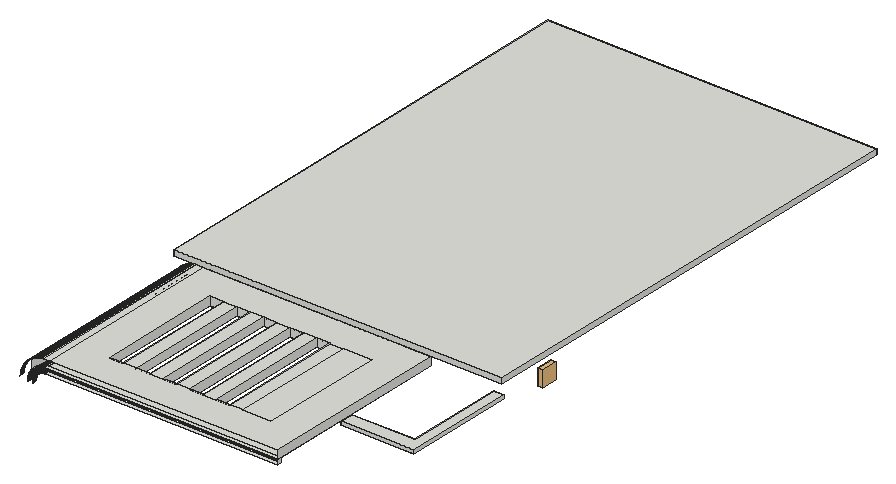
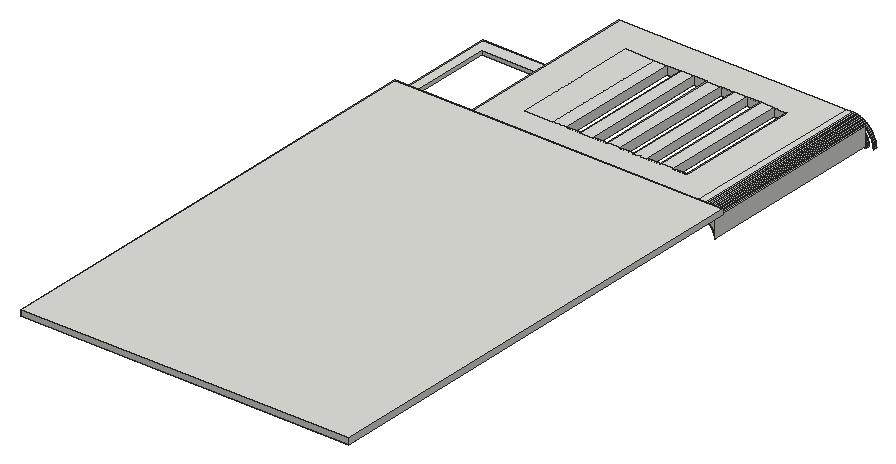
# SketchUp Ruby script. Lengths in inches.
U = 1.inch
M = Sketchup.active_model
def pt(a) = Geom::Point3d.new(a.map { |v| v * U })
def face(e, loops, mat)
  f = e.add_face(loops[0].map { |a| pt(a) })
  loops[1..].each { |l| e.add_face(l.map { |a| pt(a) }).erase! }
  f.material = f.back_material = mat if mat
  f
end
# faces: each face lists its corners as indices into pts; further lists are holes
def faces(e, pts, list, mat = nil) = list.each { |f| face(e, (f[0].is_a?(Array) ? f : [f]).map { |l| l.map { |i| pts[i] } }, mat) }
# xy, xz, yz: faces in a plane at the given z, y or x. An outline is a flat list of corners, or four numbers for a rectangle; further outlines are holes
def ring(l) = l.size == 4 ? [[l[0], l[1]], [l[2], l[1]], [l[2], l[3]], [l[0], l[3]]] : l.each_slice(2).to_a
def flat(e, list, mat, &to3) = list.each { |f| face(e, (f[0].is_a?(Array) ? f : [f]).map { |l| ring(l).map { |u, v| to3.(u, v) } }, mat) }
def xy(e, z, list, mat = nil) = flat(e, list, mat) { |x, y| [x, y, z] }
def xz(e, y, list, mat = nil) = flat(e, list, mat) { |x, z| [x, y, z] }
def yz(e, x, list, mat = nil) = flat(e, list, mat) { |y, z| [x, y, z] }
def lines(e, pts, list) = list.each { |a, b| e.add_line(pt(pts[a]), pt(pts[b])) }
# prism: a flat outline (further loops are holes) pulled along v
def prism(e, loops, v, mat = nil)
  f = face(e, loops, mat); d = Geom::Vector3d.new(v.map { |x| x * U })
  f.pushpull(f.normal.samedirection?(d) ? d.length : -d.length)
end
def box(e, o, s, mat = nil) = prism(e, [[o, [o[0] + s[0], o[1], o[2]], [o[0] + s[0], o[1] + s[1], o[2]], [o[0], o[1] + s[1], o[2]]]], [0, 0, s[2]], mat)
def at(x, y, z, deg = 0) = Geom::Transformation.translation(pt([x, y, z])) * Geom::Transformation.rotation(ORIGIN, Z_AXIS, deg.degrees)
def axes(o, x, y, z) = Geom::Transformation.new([*x, 0, *y, 0, *z, 0, *pt(o).to_a, 1])
def part(name) = M.definitions.add(name)
# library, detail: a bought-in or finely detailed component or shape, given as its bounding box
def library(name, o, s) = part(name).tap { |d| box(d.entities, o, s) }
def detail(e, o, s) = box(e.add_group.entities, o, s)
def put(e, d, t, mat = nil) = e.add_instance(d, t).tap { |i| i.material = mat if mat }
def group(e, t, mat = nil) = e.add_group.tap { |g| g.transformation = t; g.material = mat if mat }.entities
root = M.entities
c1 = library("Agrupar\#12",[-0.01,0,0],[12.55,78.74,39.39])
xy(root,358,[[27.87,40.1875,282.03,44.1875]])
xy(root,363,[[27.87,40.1875,282.03,43.1875],[27.87,43.1875,282.03,44.1875],[[27.87,44.1875,282.03,250.1875],[156.5,76.1875,171.11,214.1875],[68.83,76.1875,83.4375,214.1875],[98.05,76.1875,112.66,214.1875],[127.28,76.1875,141.89,214.1875],[185.73,76.1875,200.34,214.1875]]])
xy(root,363.89,[[27.87,40.1875,282.03,43.1875]])
xy(root,372,[[25.95,40.1875,32.83,250.1875],[[32.83,40.1875,282.03,250.1875],[68.83,76.1875,246.03,214.1875]],[83.4375,76.1875,98.05,214.1875],[112.66,76.1875,127.28,214.1875],[141.89,76.1875,156.5,214.1875],
  [171.11,76.1875,185.73,214.1875],[200.34,76.1875,214.95,214.1875],[214.95,76.1875,246.03,214.1875]])
xz(root,44.1875,[[9,344.13,9,364.72,9.02,345.61,9.02,345.02,9.01,344.72]])
xz(root,76.1875,[[68.83,363,83.4375,372],[98.05,363,112.66,372],[127.28,363,141.89,372],[156.5,363,171.11,372],[185.73,363,200.34,372]])
xz(root,214.1875,[[68.83,363,83.4375,372],[98.05,363,112.66,372],[127.28,363,141.89,372],[156.5,363,171.11,372],[185.73,363,200.34,372]])
xz(root,250.1875,[[9.02,345.02,9.02,345.61,9,364.72,9,364.73,9.39,365.09,10.0625,365.66,10.75,366.21,11.45,366.73,12.17,367.24,12.9,367.72,13.65,368.18,14.41,368.61,15.1875,369.02,15.97,369.41,16.77,369.77,17.58,370.11,18.41,370.42,19.24,370.7,20.07,370.96,20.92,371.19,21.77,371.4,22.63,371.57,23.5,371.72,24.37,371.85,25.24,371.94,25.95,372,282.03,372,282.03,363,27.87,363,27.28,362.99,26.68,362.96,26.09,362.92,25.5,362.85,24.92,362.77,24.33,362.67,23.75,362.55,23.18,362.41,22.6,362.25,22.04,362.08,21.48,361.88,20.92,361.67,20.375,361.45,19.83,361.2,19.3,360.94,18.78,360.67,18.26,360.37,17.76,360.0625,17.26,359.74,16.78,359.4,16.3,359.04,15.84,358.67,15.39,358.28,14.95,357.89,14.11,357.05,13.72,356.61,13.33,356.16,12.96,355.7,12.6,355.22,12.26,354.74,11.9375,354.24,11.63,353.74,11.33,353.22,11.06,352.7,10.8,352.17,10.55,351.625,10.33,351.08,10.12,350.52,9.92,349.96,9.75,349.4,9.59,348.82,9.45,348.25,9.33,347.67,9.23,347.08,9.15,346.5,9.08,345.91,9.04,345.32]])
yz(root,9,[[44.1875,364.72,250.1875,364.73]])
yz(root,9.02,[[44.1875,345.02,250.1875,345.61]])
yz(root,68.83,[[76.1875,363,214.1875,372]])
yz(root,83.4375,[[76.1875,363,214.1875,372]])
yz(root,98.05,[[76.1875,363,214.1875,372]])
yz(root,112.66,[[76.1875,363,214.1875,372]])
yz(root,127.28,[[76.1875,363,214.1875,372]])
yz(root,141.89,[[76.1875,363,214.1875,372]])
yz(root,156.5,[[76.1875,363,214.1875,372]])
yz(root,171.11,[[76.1875,363,214.1875,372]])
yz(root,185.73,[[76.1875,363,214.1875,372]])
yz(root,200.34,[[76.1875,363,214.1875,372]])
yz(root,282.03,[[40.1875,358,44.1875,363],[43.1875,363,250.1875,363,250.1875,372,40.1875,372,40.1875,363.89,43.1875,363.89]])
p = [[8.12,40.1875,344.75],[8.11,40.1875,344.13],[8.11,43.1875,344.13],[8.12,43.1875,344.75],[9.01,40.1875,344.72],[9,40.1875,344.13],
  [9,43.1875,344.13],[9.01,43.1875,344.72],[14.01,40.1875,344.57],[14,40.1875,344.13],[14,44.1875,344.13],[14.01,44.1875,344.57],
  [9.01,44.1875,344.72],[9,44.1875,344.13],[14.03,40.1875,345],[14.03,44.1875,345],[9.04,40.1875,345.32],[9.04,43.1875,345.32],
  [9.04,44.1875,345.32],[9.02,44.1875,345.02],[8.14,40.1875,345.37],[8.14,43.1875,345.37],[14.0625,40.1875,345.4375],[14.0625,44.1875,345.4375],
  [9.02,250.1875,345.02],[9.04,250.1875,345.32],[9.08,40.1875,345.91],[9.08,43.1875,345.91],[9.08,44.1875,345.91],[9.08,250.1875,345.91],
  [8.19,40.1875,345.99],[8.19,43.1875,345.99],[14.11,40.1875,345.87],[14.11,44.1875,345.87],[9.02,44.1875,345.61],[9,44.1875,364.72],
  [9,250.1875,364.72],[9.02,250.1875,345.61],[9.15,40.1875,346.5],[9.15,43.1875,346.5],[14.17,40.1875,346.3],[14.17,44.1875,346.3],
  [9.15,44.1875,346.5],[9.15,250.1875,346.5],[0,40.1875,346.05],[0.06,40.1875,346.76],[0.06,44.1875,346.76],[0,44.1875,346.05],
  [8.26,40.1875,346.61],[8.26,43.1875,346.61],[14.25,40.1875,346.73],[14.25,44.1875,346.73],[9.23,40.1875,347.08],[9.23,43.1875,347.08],
  [9.23,44.1875,347.08],[9.23,250.1875,347.08],[8.35,40.1875,347.22],[8.35,43.1875,347.22],[14.33,40.1875,347.16],[14.33,44.1875,347.16],
  [0.15,40.1875,347.63],[0.15,44.1875,347.63],[9.33,40.1875,347.67],[9.33,43.1875,347.67],[9.33,44.1875,347.67],[9.33,250.1875,347.67],
  [8.46,40.1875,347.83],[8.46,43.1875,347.83],[14.4375,40.1875,347.58],[14.4375,44.1875,347.58],[0.28,40.1875,348.5],[0.28,44.1875,348.5],
  [14.55,40.1875,348],[14.55,44.1875,348],[9.45,40.1875,348.25],[9.45,43.1875,348.25],[9.45,44.1875,348.25],[9.45,250.1875,348.25],
  [8.58,40.1875,348.44],[8.58,43.1875,348.44],[14.68,40.1875,348.42],[14.68,44.1875,348.42],[9.59,40.1875,348.82],[9.59,43.1875,348.82],
  [9.59,44.1875,348.82],[9.59,250.1875,348.82],[8.73,40.1875,349.05],[8.73,43.1875,349.05],[14.82,40.1875,348.83],[14.82,44.1875,348.83],
  [0.43,40.1875,349.37],[0.43,44.1875,349.37],[9.75,40.1875,349.4],[9.75,43.1875,349.4],[14.97,40.1875,349.24],[14.97,44.1875,349.24],
  [9.75,44.1875,349.4],[9.75,250.1875,349.4],[8.89,40.1875,349.64],[8.89,43.1875,349.64],[15.14,40.1875,349.64],[15.14,44.1875,349.64],
  [0.6,40.1875,350.23],[0.6,44.1875,350.23],[9.92,40.1875,349.96],[9.92,43.1875,349.96],[9.92,44.1875,349.96],[9.92,250.1875,349.96],
  [9.07,40.1875,350.24],[9.07,43.1875,350.24],[15.32,40.1875,350.04],[15.32,44.1875,350.04],[10.12,40.1875,350.52],[10.12,43.1875,350.52],
  [15.51,40.1875,350.43],[15.51,44.1875,350.43],[10.12,44.1875,350.52],[10.12,250.1875,350.52],[0.81,40.1875,351.08],[0.81,44.1875,351.08],
  [9.27,40.1875,350.83],[9.27,43.1875,350.83],[15.72,40.1875,350.8125],[15.72,44.1875,350.8125],[10.33,40.1875,351.08],[10.33,43.1875,351.08],
  [10.33,44.1875,351.08],[10.33,250.1875,351.08],[9.49,40.1875,351.41],[9.49,43.1875,351.41],[15.93,40.1875,351.19],[15.93,44.1875,351.19],
  [1.04,40.1875,351.93],[1.04,44.1875,351.93],[10.55,40.1875,351.625],[10.55,43.1875,351.625],[10.55,44.1875,351.625],[10.55,250.1875,351.625],
  [16.16,40.1875,351.5625],[16.16,44.1875,351.5625],[9.73,40.1875,351.98],[9.73,43.1875,351.98],[10.8,40.1875,352.17],[10.8,43.1875,352.17],
  [16.4,40.1875,351.93],[16.4,44.1875,351.93],[10.8,44.1875,352.17],[10.8,250.1875,352.17],[1.3,40.1875,352.76],[1.3,44.1875,352.76],
  [16.65,40.1875,352.28],[16.65,44.1875,352.28],[9.99,40.1875,352.55],[9.99,43.1875,352.55],[11.06,40.1875,352.7],[11.06,43.1875,352.7],
  [11.06,44.1875,352.7],[11.06,250.1875,352.7],[16.91,40.1875,352.63],[16.91,44.1875,352.63],[10.26,40.1875,353.1],[10.26,43.1875,353.1],
  [17.18,40.1875,352.97],[17.18,44.1875,352.97],[11.33,40.1875,353.22],[11.33,43.1875,353.22],[11.33,44.1875,353.22],[11.33,250.1875,353.22],
  [1.58,40.1875,353.59],[1.58,44.1875,353.59],[17.47,40.1875,353.3],[17.47,44.1875,353.3],[10.55,40.1875,353.65],[10.55,43.1875,353.65],
  [11.63,40.1875,353.74],[11.63,43.1875,353.74],[11.63,44.1875,353.74],[11.63,250.1875,353.74],[17.76,40.1875,353.625],[17.76,44.1875,353.625],
  [1.89,40.1875,354.42],[1.89,44.1875,354.42],[18.0625,40.1875,353.9375],[18.0625,44.1875,353.9375],[10.86,40.1875,354.19],[10.86,43.1875,354.19],
  [11.9375,40.1875,354.24],[11.9375,43.1875,354.24],[11.9375,44.1875,354.24],[11.9375,250.1875,354.24],[18.375,40.1875,354.24],[18.375,44.1875,354.24],
  [11.18,40.1875,354.72],[11.18,43.1875,354.72],[12.26,40.1875,354.74],[12.26,43.1875,354.74],[18.7,40.1875,354.53],[18.7,44.1875,354.53],
  [12.26,44.1875,354.74],[12.26,250.1875,354.74],[2.23,40.1875,355.23],[2.23,44.1875,355.23],[19.03,40.1875,354.82],[19.03,44.1875,354.82],
  [11.52,40.1875,355.24],[11.52,43.1875,355.24],[12.6,40.1875,355.22],[12.6,43.1875,355.22],[12.6,44.1875,355.22],[12.6,250.1875,355.22],
  [19.37,40.1875,355.09],[19.37,44.1875,355.09],[19.72,40.1875,355.35],[19.72,44.1875,355.35],[2.59,40.1875,356.03],[2.59,44.1875,356.03],
  [11.88,40.1875,355.75],[11.88,43.1875,355.75],[12.96,40.1875,355.7],[12.96,43.1875,355.7],[12.96,44.1875,355.7],[12.96,250.1875,355.7],
  [20.07,40.1875,355.6],[20.07,44.1875,355.6],[20.4375,40.1875,355.84],[20.4375,44.1875,355.84],[12.25,40.1875,356.24],[12.25,43.1875,356.24],
  [13.33,40.1875,356.16],[13.33,43.1875,356.16],[13.33,44.1875,356.16],[13.33,250.1875,356.16],[20.81,40.1875,356.07],[20.81,44.1875,356.07],
  [2.98,40.1875,356.8125],[2.98,44.1875,356.8125],[21.1875,40.1875,356.28],[21.1875,44.1875,356.28],[12.64,40.1875,356.73],[12.64,43.1875,356.73],
  [13.72,40.1875,356.61],[13.72,43.1875,356.61],[13.72,44.1875,356.61],[13.72,250.1875,356.61],[21.57,40.1875,356.49],[21.57,44.1875,356.49],
  [21.96,40.1875,356.68],[21.96,44.1875,356.68],[14.11,40.1875,357.05],[14.11,43.1875,357.05],[14.11,44.1875,357.05],[14.11,250.1875,357.05],
  [13.04,40.1875,357.2],[13.04,43.1875,357.2],[22.36,40.1875,356.86],[22.36,44.1875,356.86],[3.39,40.1875,357.59],[3.39,44.1875,357.59],
  [22.76,40.1875,357.03],[22.76,44.1875,357.03],[14.53,40.1875,357.47],[14.53,43.1875,357.47],[23.17,40.1875,357.18],[23.17,44.1875,357.18],
  [14.53,44.1875,357.47],[14.53,250.1875,357.47],[13.46,40.1875,357.66],[13.46,43.1875,357.66],[23.58,40.1875,357.32],[23.58,44.1875,357.32],
  [24,40.1875,357.45],[24,44.1875,357.45],[24.42,40.1875,357.5625],[24.42,44.1875,357.5625],[14.95,40.1875,357.89],[14.95,43.1875,357.89],
  [14.95,44.1875,357.89],[14.95,250.1875,357.89],[3.82,40.1875,358.35],[3.82,44.1875,358.35],[24.84,40.1875,357.67],[24.84,44.1875,357.67],
  [13.89,40.1875,358.11],[13.89,43.1875,358.11],[25.27,40.1875,357.75],[25.27,44.1875,357.75],[25.7,40.1875,357.83],[25.7,44.1875,357.83],
  [26.13,40.1875,357.89],[26.13,44.1875,357.89],[15.39,40.1875,358.28],[15.39,43.1875,358.28],[26.5625,40.1875,357.9375],[26.5625,44.1875,357.9375],
  [27,40.1875,357.97],[27,44.1875,357.97],[15.39,44.1875,358.28],[15.39,250.1875,358.28],[27.43,40.1875,357.99],[27.43,44.1875,357.99],
  [27.87,40.1875,358],[27.87,44.1875,358],[14.34,40.1875,358.54],[14.34,43.1875,358.54],[15.84,40.1875,358.67],[15.84,43.1875,358.67],
  [15.84,44.1875,358.67],[15.84,250.1875,358.67],[4.28,40.1875,359.1],[4.28,44.1875,359.1],[14.8,40.1875,358.96],[14.8,43.1875,358.96],
  [16.3,40.1875,359.04],[16.3,43.1875,359.04],[16.3,44.1875,359.04],[16.3,250.1875,359.04],[15.27,40.1875,359.36],[15.27,43.1875,359.36],
  [16.78,40.1875,359.4],[16.78,43.1875,359.4],[16.78,44.1875,359.4],[16.78,250.1875,359.4],[4.76,40.1875,359.83],[4.76,44.1875,359.83],
  [15.76,40.1875,359.75],[15.76,43.1875,359.75],[17.26,40.1875,359.74],[17.26,43.1875,359.74],[17.26,44.1875,359.74],[17.26,250.1875,359.74],
  [16.25,40.1875,360.12],[16.25,43.1875,360.12],[17.76,40.1875,360.0625],[17.76,43.1875,360.0625],[17.76,44.1875,360.0625],[17.76,250.1875,360.0625],
  [5.27,40.1875,360.55],[5.27,44.1875,360.55],[16.76,40.1875,360.48],[16.76,43.1875,360.48],[18.26,40.1875,360.37],[18.26,43.1875,360.37],
  [18.26,44.1875,360.37],[18.26,250.1875,360.37],[18.78,40.1875,360.67],[18.78,43.1875,360.67],[18.78,44.1875,360.67],[18.78,250.1875,360.67],
  [17.28,40.1875,360.82],[17.28,43.1875,360.82],[5.79,40.1875,361.25],[5.79,44.1875,361.25],[19.3,40.1875,360.94],[19.3,43.1875,360.94],
  [19.3,44.1875,360.94],[19.3,250.1875,360.94],[17.81,40.1875,361.14],[17.81,43.1875,361.14],[19.83,40.1875,361.2],[19.83,43.1875,361.2],
  [19.83,44.1875,361.2],[19.83,250.1875,361.2],[18.35,40.1875,361.45],[18.35,43.1875,361.45],[20.375,40.1875,361.45],[20.375,43.1875,361.45],
  [20.375,44.1875,361.45],[20.375,250.1875,361.45],[6.34,40.1875,361.9375],[6.34,44.1875,361.9375],[18.9,40.1875,361.74],[18.9,43.1875,361.74],
  [20.92,40.1875,361.67],[20.92,43.1875,361.67],[20.92,44.1875,361.67],[20.92,250.1875,361.67],[19.45,40.1875,362.01],[19.45,43.1875,362.01],
  [21.48,40.1875,361.88],[21.48,43.1875,361.88],[21.48,44.1875,361.88],[21.48,250.1875,361.88],[6.91,40.1875,362.61],[6.91,44.1875,362.61],
  [22.04,40.1875,362.08],[22.04,43.1875,362.08],[22.04,44.1875,362.08],[22.04,250.1875,362.08],[20.02,40.1875,362.27],[20.02,43.1875,362.27],
  [22.6,40.1875,362.25],[22.6,43.1875,362.25],[22.6,44.1875,362.25],[22.6,250.1875,362.25],[20.59,40.1875,362.51],[20.59,43.1875,362.51],
  [23.18,40.1875,362.41],[23.18,43.1875,362.41],[23.18,44.1875,362.41],[23.18,250.1875,362.41],[23.75,40.1875,362.55],[23.75,43.1875,362.55],
  [23.75,44.1875,362.55],[23.75,250.1875,362.55],[21.17,40.1875,362.73],[21.17,43.1875,362.73],[24.33,40.1875,362.67],[24.33,43.1875,362.67],
  [24.33,44.1875,362.67],[24.33,250.1875,362.67],[7.5,40.1875,363.26],[7.5,44.1875,363.26],[21.76,40.1875,362.93],[21.76,43.1875,362.93],
  [24.92,40.1875,362.77],[24.92,43.1875,362.77],[24.92,44.1875,362.77],[24.92,250.1875,362.77],[25.5,40.1875,362.85],[25.5,43.1875,362.85],
  [25.5,44.1875,362.85],[25.5,250.1875,362.85],[22.36,40.1875,363.11],[22.36,43.1875,363.11],[26.09,40.1875,362.92],[26.09,43.1875,362.92],
  [26.68,40.1875,362.96],[26.68,43.1875,362.96],[26.09,44.1875,362.92],[26.68,44.1875,362.96],[26.09,250.1875,362.92],[26.68,250.1875,362.96],
  [27.28,40.1875,362.99],[27.28,43.1875,362.99],[27.87,40.1875,363],[27.87,43.1875,363],[27.28,44.1875,362.99],[27.87,44.1875,363],
  [27.28,250.1875,362.99],[27.87,250.1875,363],[22.95,40.1875,363.27],[22.95,43.1875,363.27],[8.11,40.1875,363.89],[8.11,44.1875,363.89],
  [23.56,40.1875,363.42],[23.56,43.1875,363.42],[24.17,40.1875,363.54],[24.17,43.1875,363.54],[24.78,40.1875,363.65],[24.78,43.1875,363.65],
  [25.39,40.1875,363.74],[25.39,43.1875,363.74],[26.01,40.1875,363.81],[26.01,43.1875,363.81],[26.63,40.1875,363.86],[26.63,43.1875,363.86],
  [8.74,40.1875,364.5],[8.74,44.1875,364.5],[27.25,40.1875,363.88],[27.25,43.1875,363.88],[27.87,40.1875,363.89],[27.87,43.1875,363.89],
  [9.39,40.1875,365.09],[9.39,250.1875,365.09],[9,250.1875,364.73],[9,44.1875,364.73],[10.0625,40.1875,365.66],[10.0625,250.1875,365.66],
  [10.75,40.1875,366.21],[10.75,250.1875,366.21],[11.45,40.1875,366.73],[11.45,250.1875,366.73],[12.17,40.1875,367.24],[12.17,250.1875,367.24],
  [12.9,40.1875,367.72],[12.9,250.1875,367.72],[13.65,40.1875,368.18],[13.65,250.1875,368.18],[14.41,40.1875,368.61],[14.41,250.1875,368.61],
  [15.1875,40.1875,369.02],[15.1875,250.1875,369.02],[15.97,40.1875,369.41],[15.97,250.1875,369.41],[16.77,40.1875,369.77],[16.77,250.1875,369.77],
  [17.58,40.1875,370.11],[17.58,250.1875,370.11],[18.41,40.1875,370.42],[18.41,250.1875,370.42],[19.24,40.1875,370.7],[19.24,250.1875,370.7],
  [20.07,40.1875,370.96],[20.07,250.1875,370.96],[20.92,40.1875,371.19],[20.92,250.1875,371.19],[21.77,40.1875,371.4],[21.77,250.1875,371.4],
  [22.63,40.1875,371.57],[22.63,250.1875,371.57],[23.5,40.1875,371.72],[23.5,250.1875,371.72],[24.37,40.1875,371.85],[24.37,250.1875,371.85],
  [25.24,40.1875,371.94],[25.24,250.1875,371.94],[25.95,40.1875,372],[25.95,250.1875,372]]
faces(root,p,[[0,1,2,3],[4,5,6,7],[8,9,10,11],[12,7,6,13],[14,8,11,15],[16,4,7,17],[18,17,7,12,19],[20,0,3,21],
  [22,14,15,23],[19,24,25,18],[26,16,17,27],[28,27,17,18],[29,28,18,25],[30,20,21,31],[32,22,23,33],[34,35,36,37],
  [38,26,27,39],[40,32,33,41],[42,39,27,28],[43,42,28,29],[44,45,46,47],[48,30,31,49],[50,40,41,51],[52,38,39,53],
  [54,53,39,42],[55,54,42,43],[56,48,49,57],[58,50,51,59],[45,60,61,46],[62,52,53,63],[64,63,53,54],[65,64,54,55],
  [66,56,57,67],[68,58,59,69],[60,70,71,61],[72,68,69,73],[74,62,63,75],[76,75,63,64],[77,76,64,65],[78,66,67,79],
  [80,72,73,81],[82,74,75,83],[84,83,75,76],[85,84,76,77],[86,78,79,87],[88,80,81,89],[70,90,91,71],[92,82,83,93],
  [94,88,89,95],[96,93,83,84],[97,96,84,85],[98,86,87,99],[100,94,95,101],[90,102,103,91],[104,92,93,105],[106,105,93,96],
  [107,106,96,97],[108,98,99,109],[110,100,101,111],[112,104,105,113],[114,110,111,115],[116,113,105,106],[117,116,106,107],[102,118,119,103],
  [120,108,109,121],[122,114,115,123],[124,112,113,125],[126,125,113,116],[127,126,116,117],[128,120,121,129],[130,122,123,131],[118,132,133,119],
  [134,124,125,135],[136,135,125,126],[137,136,126,127],[138,130,131,139],[140,128,129,141],[142,134,135,143],[144,138,139,145],[146,143,135,136],
  [147,146,136,137],[132,148,149,133],[150,144,145,151],[152,140,141,153],[154,142,143,155],[156,155,143,146],[157,156,146,147],[158,150,151,159],
  [160,152,153,161],[162,158,159,163],[164,154,155,165],[166,165,155,156],[167,166,156,157],[148,168,169,149],[170,162,163,171],[172,160,161,173],
  [174,164,165,175],[176,175,165,166],[177,176,166,167],[178,170,171,179],[168,180,181,169],[182,178,179,183],[184,172,173,185],[186,174,175,187],
  [188,187,175,176],[189,188,176,177],[190,182,183,191],[192,184,185,193],[194,186,187,195],[196,190,191,197],[198,195,187,188],[199,198,188,189],
  [180,200,201,181],[202,196,197,203],[204,192,193,205],[206,194,195,207],[208,207,195,198],[209,208,198,199],[210,202,203,211],[212,210,211,213],
  [200,214,215,201],[216,204,205,217],[218,206,207,219],[220,219,207,208],[221,220,208,209],[222,212,213,223],[224,222,223,225],[226,216,217,227],
  [228,218,219,229],[230,229,219,220],[231,230,220,221],[232,224,225,233],[214,234,235,215],[236,232,233,237],[238,226,227,239],[240,228,229,241],
  [242,241,229,230],[243,242,230,231],[244,236,237,245],[246,244,245,247],[248,240,241,249],[250,249,241,242],[251,250,242,243],[252,238,239,253],
  [254,246,247,255],[234,256,257,235],[258,254,255,259],[260,248,249,261],[262,258,259,263],[264,261,249,250],[265,264,250,251],[266,252,253,267],
  [268,262,263,269],[270,268,269,271],[272,270,271,273],[274,260,261,275],[276,275,261,264],[277,276,264,265],[256,278,279,257],[280,272,273,281],
  [282,266,267,283],[284,280,281,285],[286,284,285,287],[288,286,287,289],[290,274,275,291],[292,288,289,293],[294,292,293,295],[296,291,275,276],
  [297,296,276,277],[298,294,295,299],[300,298,299,301],[302,282,283,303],[304,290,291,305],[306,305,291,296],[307,306,296,297],[278,308,309,279],
  [310,302,303,311],[312,304,305,313],[314,313,305,306],[315,314,306,307],[316,310,311,317],[318,312,313,319],[320,319,313,314],[321,320,314,315],
  [308,322,323,309],[324,316,317,325],[326,318,319,327],[328,327,319,320],[329,328,320,321],[330,324,325,331],[332,326,327,333],[334,333,327,328],
  [335,334,328,329],[322,336,337,323],[338,330,331,339],[340,332,333,341],[342,341,333,334],[343,342,334,335],[344,340,341,345],[346,345,341,342],
  [347,346,342,343],[348,338,339,349],[336,350,351,337],[352,344,345,353],[354,353,345,346],[355,354,346,347],[356,348,349,357],[358,352,353,359],
  [360,359,353,354],[361,360,354,355],[362,356,357,363],[364,358,359,365],[366,365,359,360],[367,366,360,361],[350,368,369,351],[370,362,363,371],
  [372,364,365,373],[374,373,365,366],[375,374,366,367],[376,370,371,377],[378,372,373,379],[380,379,373,374],[381,380,374,375],[368,382,383,369],
  [384,378,379,385],[386,385,379,380],[387,386,380,381],[388,376,377,389],[390,384,385,391],[392,391,385,386],[393,392,386,387],[394,388,389,395],
  [396,390,391,397],[398,397,391,392],[399,398,392,393],[400,396,397,401],[402,401,397,398],[403,402,398,399],[404,394,395,405],[406,400,401,407],
  [408,407,401,402],[409,408,402,403],[382,410,411,383],[412,404,405,413],[414,406,407,415],[416,415,407,408],[417,416,408,409],[418,414,415,419],
  [420,419,415,416],[421,420,416,417],[422,412,413,423],[424,418,419,425],[426,424,425,427],[428,425,419,420],[429,427,425,428],[430,428,420,421],
  [431,429,428,430],[432,426,427,433],[434,432,433,435],[436,433,427,429],[437,435,433,436],[438,436,429,431],[439,437,436,438],[440,422,423,441],
  [410,442,443,411],[444,440,441,445],[446,444,445,447],[448,446,447,449],[450,448,449,451],[452,450,451,453],[454,452,453,455],[442,456,457,443],
  [458,454,455,459],[460,458,459,461],[456,462,463,464,465,457],[462,466,467,463],[466,468,469,467],[468,470,471,469],[470,472,473,471],[472,474,475,473],
  [474,476,477,475],[476,478,479,477],[478,480,481,479],[480,482,483,481],[482,484,485,483],[484,486,487,485],[486,488,489,487],[488,490,491,489],
  [490,492,493,491],[492,494,495,493],[494,496,497,495],[496,498,499,497],[498,500,501,499],[500,502,503,501],[502,504,505,503],[504,506,507,505]])
put(root,c1,axes([364.97,318.42,348],[-0.45,0,0],[0,-0.2286,0],[0,0,0.45697]))
g1 = group(root,at(282.53,127.1875,358.51))
prism(g1,[[[79.53,0,0],[-0.5,0,0],[-0.5,15,0],[68.53,15,0],[68.53,123,0],[79.53,123,0]]],[0,0,4])
g2 = group(root,at(0,250.1875,372))
box(g2,[0,0,0],[360.05,513,6])
